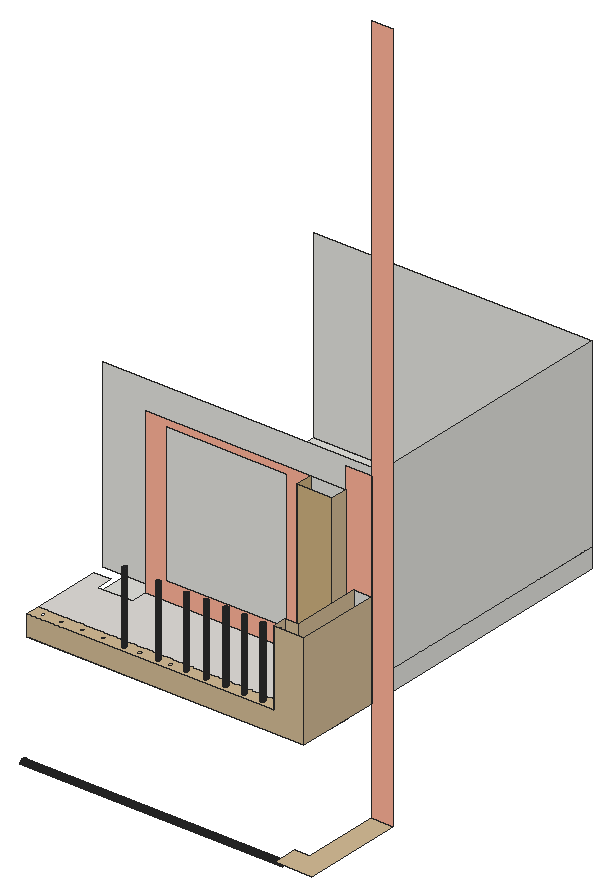
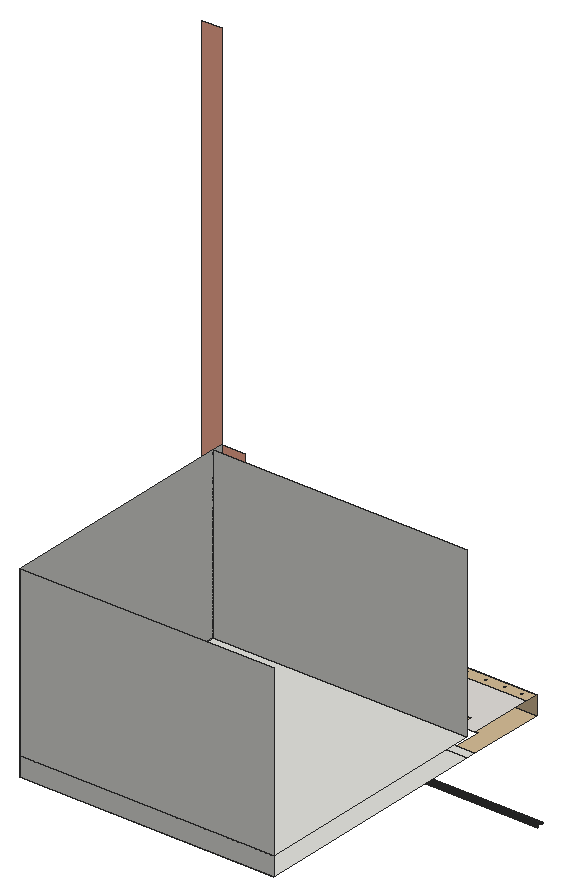
# SketchUp Ruby script. Lengths in inches.
U = 1.inch
M = Sketchup.active_model
def pt(a) = Geom::Point3d.new(a.map { |v| v * U })
def face(e, loops, mat)
  f = e.add_face(loops[0].map { |a| pt(a) })
  loops[1..].each { |l| e.add_face(l.map { |a| pt(a) }).erase! }
  f.material = f.back_material = mat if mat
  f
end
# faces: each face lists its corners as indices into pts; further lists are holes
def faces(e, pts, list, mat = nil) = list.each { |f| face(e, (f[0].is_a?(Array) ? f : [f]).map { |l| l.map { |i| pts[i] } }, mat) }
# xy, xz, yz: faces in a plane at the given z, y or x. An outline is a flat list of corners, or four numbers for a rectangle; further outlines are holes
def ring(l) = l.size == 4 ? [[l[0], l[1]], [l[2], l[1]], [l[2], l[3]], [l[0], l[3]]] : l.each_slice(2).to_a
def flat(e, list, mat, &to3) = list.each { |f| face(e, (f[0].is_a?(Array) ? f : [f]).map { |l| ring(l).map { |u, v| to3.(u, v) } }, mat) }
def xy(e, z, list, mat = nil) = flat(e, list, mat) { |x, y| [x, y, z] }
def xz(e, y, list, mat = nil) = flat(e, list, mat) { |x, z| [x, y, z] }
def yz(e, x, list, mat = nil) = flat(e, list, mat) { |y, z| [x, y, z] }
def lines(e, pts, list) = list.each { |a, b| e.add_line(pt(pts[a]), pt(pts[b])) }
# prism: a flat outline (further loops are holes) pulled along v
def prism(e, loops, v, mat = nil)
  f = face(e, loops, mat); d = Geom::Vector3d.new(v.map { |x| x * U })
  f.pushpull(f.normal.samedirection?(d) ? d.length : -d.length)
end
def box(e, o, s, mat = nil) = prism(e, [[o, [o[0] + s[0], o[1], o[2]], [o[0] + s[0], o[1] + s[1], o[2]], [o[0], o[1] + s[1], o[2]]]], [0, 0, s[2]], mat)
def at(x, y, z, deg = 0) = Geom::Transformation.translation(pt([x, y, z])) * Geom::Transformation.rotation(ORIGIN, Z_AXIS, deg.degrees)
def axes(o, x, y, z) = Geom::Transformation.new([*x, 0, *y, 0, *z, 0, *pt(o).to_a, 1])
def part(name) = M.definitions.add(name)
# library, detail: a bought-in or finely detailed component or shape, given as its bounding box
def library(name, o, s) = part(name).tap { |d| box(d.entities, o, s) }
def detail(e, o, s) = box(e.add_group.entities, o, s)
def put(e, d, t, mat = nil) = e.add_instance(d, t).tap { |i| i.material = mat if mat }
def group(e, t, mat = nil) = e.add_group.tap { |g| g.transformation = t; g.material = mat if mat }.entities
root = M.entities
M.materials.add("[Color B02]").color = [255, 178, 153]
M.materials.add("[Formica Beige]").color = [211, 187, 149]
M.materials.add("[Formica Laminate Dark]").color = [50, 53, 60]
M.materials.add("[Terrazzo Tile Accent]").color = [224, 221, 217]
M.materials.add("[Wood Floor Light]").color = [204, 176, 127]
xy(root,185.07,[[687.39,128.83,687.78,128.89,688.14,129.04,688.45,129.27,688.6875,129.58,688.84,129.95,688.89,130.33,688.84,130.72,688.6875,131.08,688.45,131.4,688.14,131.63,687.78,131.78,687.39,131.83,687,131.78,686.64,131.63,686.33,131.4,686.09,131.08,685.9375,130.72,685.89,130.33,685.9375,129.95,686.09,129.58,686.33,129.27,686.64,129.04,687,128.89]])
xy(root,189,[[765.67,122.79,786.87,122.79,786.87,182.57,774.15,182.57,774.15,137.11,765.67,137.11]],"[Formica Beige]")
xy(root,236.59,[[741.45,165.2,760.39,182.57]])
xy(root,236.59,[[641.83,165.2,741.45,182.57]],"[Wood Floor Light]")
xy(root,249,[[641.83,165.2,741.45,182.57],[741.45,165.2,760.39,182.57],[611.125,182.57,774.15,189.24],[611.125,189.24,774.15,344.36]])
xy(root,249,[[611.125,133.3,611.125,182.57,622.89,182.57,622.89,165.2,760.39,165.2,760.39,182.57,774.15,182.57,774.15,133.3]],"[Formica Beige]")
xy(root,261,[[665.36,136.16,665.06,136.2,664.77,136.32,664.52,136.51,664.34,136.76,664.22,137.04,664.18,137.35,664.22,137.66,664.34,137.94,664.52,138.19,664.77,138.38,665.06,138.5,665.36,138.54,665.67,138.5,665.96,138.38,666.2,138.19,666.39,137.94,666.51,137.66,666.55,137.35,666.51,137.04,666.39,136.76,666.2,136.51,665.96,136.32,665.67,136.2],[684.99,136.16,684.68,136.2,684.4,136.32,684.15,136.51,683.96,136.76,683.84,137.04,683.8,137.35,683.84,137.66,683.96,137.94,684.15,138.19,684.4,138.38,684.68,138.5,684.99,138.54,685.3,138.5,685.58,138.38,685.83,138.19,686.02,137.94,686.14,137.66,686.18,137.35,686.14,137.04,686.02,136.76,685.83,136.51,685.58,136.32,685.3,136.2],[701.43,136.16,701.12,136.2,700.83,136.32,700.59,136.51,700.4,136.76,700.28,137.04,700.24,137.35,700.28,137.66,700.4,137.94,700.59,138.19,700.83,138.38,701.12,138.5,701.43,138.54,701.73,138.5,702.02,138.38,702.27,138.19,702.46,137.94,702.57,137.66,702.61,137.35,702.57,137.04,702.46,136.76,702.27,136.51,702.02,136.32,701.73,136.2],[713.18,136.16,712.87,136.2,712.58,136.32,712.34,136.51,712.15,136.76,712.03,137.04,711.99,137.35,712.03,137.66,712.15,137.94,712.34,138.19,712.58,138.38,712.87,138.5,713.18,138.54,713.48,138.5,713.77,138.38,714.02,138.19,714.21,137.94,714.32,137.66,714.36,137.35,714.32,137.04,714.21,136.76,714.02,136.51,713.77,136.32,713.48,136.2],[724.8,136.16,724.49,136.2,724.21,136.32,723.96,136.51,723.77,136.76,723.66,137.04,723.61,137.35,723.66,137.66,723.77,137.94,723.96,138.19,724.21,138.38,724.49,138.5,724.8,138.54,725.11,138.5,725.4,138.38,725.64,138.19,725.83,137.94,725.95,137.66,725.99,137.35,725.95,137.04,725.83,136.76,725.64,136.51,725.4,136.32,725.11,136.2],
  [735.74,136.16,735.43,136.2,735.15,136.32,734.9,136.51,734.71,136.76,734.59,137.04,734.55,137.35,734.59,137.66,734.71,137.94,734.9,138.19,735.15,138.38,735.43,138.5,735.74,138.54,736.05,138.5,736.33,138.38,736.58,138.19,736.77,137.94,736.89,137.66,736.93,137.35,736.89,137.04,736.77,136.76,736.58,136.51,736.33,136.32,736.05,136.2],[746.55,136.16,746.24,136.2,745.96,136.32,745.71,136.51,745.52,136.76,745.41,137.04,745.36,137.35,745.41,137.66,745.52,137.94,745.71,138.19,745.96,138.38,746.24,138.5,746.55,138.54,746.86,138.5,747.15,138.38,747.39,138.19,747.58,137.94,747.7,137.66,747.74,137.35,747.7,137.04,747.58,136.76,747.39,136.51,747.15,136.32,746.86,136.2],[738.55,172.64,758.88,182.57],[611.125,189.24,774.15,344.36]])
xy(root,261,[[[611.125,133.3,755.9375,141.82],[692.47,135.92,692.13,135.96,691.82,136.09,691.55,136.3,691.34,136.57,691.21,136.89,691.16,137.23,691.21,137.57,691.34,137.88,691.55,138.16,691.82,138.36,692.13,138.5,692.47,138.54,692.8125,138.5,693.13,138.36,693.4,138.16,693.61,137.88,693.74,137.57,693.79,137.23,693.74,136.89,693.61,136.57,693.4,136.3,693.13,136.09,692.8125,135.96],[674.41,135.92,674.07,135.96,673.75,136.09,673.48,136.3,673.27,136.57,673.14,136.89,673.1,137.23,673.14,137.57,673.27,137.88,673.48,138.16,673.75,138.36,674.07,138.5,674.41,138.54,674.75,138.5,675.07,138.36,675.34,138.16,675.55,137.88,675.68,137.57,675.72,137.23,675.68,136.89,675.55,136.57,675.34,136.3,675.07,136.09,674.75,135.96],[617.36,136.16,617.06,136.2,616.77,136.32,616.52,136.51,616.34,136.76,616.22,137.04,616.18,137.35,616.22,137.66,616.34,137.94,616.52,138.19,616.77,138.38,617.06,138.5,617.36,138.54,617.67,138.5,617.96,138.38,618.2,138.19,618.39,137.94,618.51,137.66,618.55,137.35,618.51,137.04,618.39,136.76,618.2,136.51,617.96,136.32,617.67,136.2],[735.74,136.16,735.43,136.2,735.15,136.32,734.9,136.51,734.71,136.76,734.59,137.04,734.55,137.35,734.59,137.66,734.71,137.94,734.9,138.19,735.15,138.38,735.43,138.5,735.74,138.54,736.05,138.5,736.33,138.38,736.58,138.19,736.77,137.94,736.89,137.66,736.93,137.35,736.89,137.04,736.77,136.76,736.58,136.51,736.33,136.32,736.05,136.2],[628.3,136.16,627.99,136.2,627.71,136.32,627.46,136.51,627.27,136.76,627.16,137.04,627.11,137.35,627.16,137.66,627.27,137.94,627.46,138.19,627.71,138.38,627.99,138.5,628.3,138.54,628.61,138.5,628.9,138.38,629.14,138.19,629.33,137.94,629.45,137.66,629.49,137.35,629.45,137.04,629.33,136.76,629.14,136.51,628.9,136.32,628.61,136.2],[724.8,136.16,724.49,136.2,724.21,136.32,723.96,136.51,723.77,136.76,723.66,137.04,723.61,137.35,723.66,137.66,723.77,137.94,723.96,138.19,724.21,138.38,724.49,138.5,724.8,138.54,725.11,138.5,725.4,138.38,725.64,138.19,725.83,137.94,725.95,137.66,725.99,137.35,725.95,137.04,725.83,136.76,725.64,136.51,725.4,136.32,725.11,136.2],[640.36,136.16,640.06,136.2,639.77,136.32,639.52,136.51,639.34,136.76,639.22,137.04,639.18,137.35,639.22,137.66,639.34,137.94,639.52,138.19,639.77,138.38,640.06,138.5,640.36,138.54,640.67,138.5,640.96,138.38,641.2,138.19,641.39,137.94,641.51,137.66,641.55,137.35,641.51,137.04,641.39,136.76,641.2,136.51,640.96,136.32,640.67,136.2],[713.18,136.16,712.87,136.2,712.58,136.32,712.34,136.51,712.15,136.76,712.03,137.04,711.99,137.35,712.03,137.66,712.15,137.94,712.34,138.19,712.58,138.38,712.87,138.5,713.18,138.54,713.48,138.5,713.77,138.38,714.02,138.19,714.21,137.94,714.32,137.66,714.36,137.35,714.32,137.04,714.21,136.76,714.02,136.51,713.77,136.32,713.48,136.2],[652.55,136.16,652.24,136.2,651.96,136.32,651.71,136.51,651.52,136.76,651.41,137.04,651.36,137.35,651.41,137.66,651.52,137.94,651.71,138.19,651.96,138.38,652.24,138.5,652.55,138.54,652.86,138.5,653.15,138.38,653.39,138.19,653.58,137.94,653.7,137.66,653.74,137.35,653.7,137.04,653.58,136.76,653.39,136.51,653.15,136.32,652.86,136.2],[701.43,136.16,701.12,136.2,700.83,136.32,700.59,136.51,700.4,136.76,700.28,137.04,700.24,137.35,700.28,137.66,700.4,137.94,700.59,138.19,700.83,138.38,701.12,138.5,701.43,138.54,701.73,138.5,702.02,138.38,702.27,138.19,702.46,137.94,702.57,137.66,702.61,137.35,702.57,137.04,702.46,136.76,702.27,136.51,702.02,136.32,701.73,136.2],[665.36,136.16,665.06,136.2,664.77,136.32,664.52,136.51,664.34,136.76,664.22,137.04,664.18,137.35,664.22,137.66,664.34,137.94,664.52,138.19,664.77,138.38,665.06,138.5,665.36,138.54,665.67,138.5,665.96,138.38,666.2,138.19,666.39,137.94,666.51,137.66,666.55,137.35,666.51,137.04,666.39,136.76,666.2,136.51,665.96,136.32,665.67,136.2],[684.99,136.16,684.68,136.2,684.4,136.32,684.15,136.51,683.96,136.76,683.84,137.04,683.8,137.35,683.84,137.66,683.96,137.94,684.15,138.19,684.4,138.38,684.68,138.5,684.99,138.54,685.3,138.5,685.58,138.38,685.83,138.19,686.02,137.94,686.14,137.66,686.18,137.35,686.14,137.04,686.02,136.76,685.83,136.51,685.58,136.32,685.3,136.2],[746.55,136.16,746.24,136.2,745.96,136.32,745.71,136.51,745.52,136.76,745.41,137.04,745.36,137.35,745.41,137.66,745.52,137.94,745.71,138.19,745.96,138.38,746.24,138.5,746.55,138.54,746.86,138.5,747.15,138.38,747.39,138.19,747.58,137.94,747.7,137.66,747.74,137.35,747.7,137.04,747.58,136.76,747.39,136.51,747.15,136.32,746.86,136.2]]],"[Formica Beige]")
xy(root,261,[[611.125,141.82,764,141.82,764,182.57,758.88,182.57,758.88,172.64,738.55,172.64,738.55,182.57,641.63,182.57,641.63,172.64,621.3,172.64,621.3,182.57,611.125,182.57]],"[Terrazzo Tile Accent]")
xz(root,133.3,[[611.125,249,774.15,249,774.15,305.625,755.9375,305.625,755.9375,261,611.125,261]],"[Formica Beige]")
xz(root,141.82,[[755.9375,261,764,305.625]],"[Formica Beige]")
xz(root,165.2,[[641.83,236.59,741.45,249],[741.45,236.59,760.39,249]],"[Wood Floor Light]")
xz(root,172.64,[[738.55,261,758.88,356.625]],"[Wood Floor Light]")
xz(root,182.57,[[641.83,236.59,741.45,249],[741.45,236.59,760.39,249],[738.55,261,758.88,356.625]])
xz(root,182.57,[[774.15,189,786.87,609],[[641.63,261,738.55,356.625],[653.42,271.33,724.17,352.83]],[758.88,261,764,261,764,305.625,774.15,305.625,774.15,369,758.88,369]],"[Color B02]")
xz(root,189.24,[[611.125,261,774.15,369]])
xz(root,344.36,[[611.125,249,774.15,261],[611.125,261,774.15,369]])
yz(root,738.55,[[172.64,261,182.57,356.625]],"[Wood Floor Light]")
yz(root,741.45,[[165.2,236.59,182.57,249]])
yz(root,755.9375,[[[133.3,261,141.82,305.625],[138.08,300.72,138.39,300.77,138.68,300.88,138.92,301.07,139.11,301.32,139.23,301.6,139.27,301.91,139.23,302.22,139.11,302.51,138.92,302.75,138.68,302.94,138.39,303.06,138.08,303.1,137.78,303.06,137.49,302.94,137.25,302.75,137.06,302.51,136.9375,302.22,136.9,301.91,136.9375,301.6,137.06,301.32,137.25,301.07,137.49,300.88,137.78,300.77]]],"[Formica Beige]")
yz(root,758.88,[[172.64,261,182.57,356.625]],"[Formica Beige]")
yz(root,760.39,[[165.2,236.59,182.57,249]],"[Wood Floor Light]")
yz(root,764,[[141.82,261,182.57,305.625]],"[Formica Beige]")
yz(root,774.15,[[182.57,249,189.24,369],[189.24,249,344.36,261],[189.24,261,344.36,369]])
yz(root,774.15,[[133.3,249,182.57,305.625]],"[Formica Beige]")
p = [[765.67,128.24,184.07],[765.67,128.3125,184.59],[611.125,128.3125,184.59],[611.125,128.24,184.07],[765.67,132.18,184.59],[765.67,132.24,184.07],
  [611.125,132.24,184.07],[611.125,132.18,184.59],[765.67,128.51,185.07],[611.125,128.51,185.07],[765.67,131.98,185.07],[611.125,131.98,185.07],
  [765.67,128.83,185.49],[611.125,128.83,185.49],[765.67,131.66,185.49],[611.125,131.66,185.49],[765.67,129.24,185.8],[611.125,129.24,185.8],
  [765.67,131.24,185.8],[611.125,131.24,185.8],[765.67,129.73,186],[611.125,129.73,186],[765.67,130.76,186],[611.125,130.76,186],
  [765.67,130.24,186.07],[611.125,130.24,186.07],[664.77,136.32,261],[665.06,136.2,261],[665.06,136.2,302.8125],[664.77,136.32,302.8125],
  [665.36,136.16,261],[665.36,136.16,302.8125],[665.67,136.2,261],[665.67,136.2,302.8125],[665.96,136.32,261],[665.96,136.32,302.8125],
  [684.4,136.32,261],[684.68,136.2,261],[684.68,136.2,302.125],[684.4,136.32,302.125],[684.99,136.16,261],[684.99,136.16,302.125],
  [685.3,136.2,261],[685.3,136.2,302.125],[685.58,136.32,261],[685.58,136.32,302.125],[700.83,136.32,261],[701.12,136.2,261],
  [701.12,136.2,301.9375],[700.83,136.32,301.9375],[701.43,136.16,261],[701.43,136.16,301.9375],[701.73,136.2,261],[701.73,136.2,301.9375],
  [702.02,136.32,261],[702.02,136.32,301.9375],[712.58,136.32,261],[712.87,136.2,261],[712.87,136.2,302.3125],[712.58,136.32,302.3125],
  [713.18,136.16,261],[713.18,136.16,302.3125],[713.48,136.2,261],[713.48,136.2,302.3125],[713.77,136.32,261],[713.77,136.32,302.3125],
  [724.21,136.32,261],[724.49,136.2,261],[724.49,136.2,302.375],[724.21,136.32,302.375],[724.8,136.16,261],[724.8,136.16,302.375],
  [725.11,136.2,261],[725.11,136.2,302.375],[725.4,136.32,261],[725.4,136.32,302.375],[735.15,136.32,261],[735.43,136.2,261],
  [735.43,136.2,302.1875],[735.15,136.32,302.1875],[735.74,136.16,261],[735.74,136.16,302.1875],[736.05,136.2,261],[736.05,136.2,302.1875],
  [736.33,136.32,261],[736.33,136.32,302.1875],[745.96,136.32,261],[746.24,136.2,261],[746.24,136.2,301.875],[745.96,136.32,301.875],
  [746.55,136.16,261],[746.55,136.16,301.875],[746.86,136.2,261],[746.86,136.2,301.875],[747.15,136.32,261],[747.15,136.32,301.875],
  [664.52,136.51,261],[664.52,136.51,302.8125],[666.2,136.51,261],[666.2,136.51,302.8125],[684.15,136.51,261],[684.15,136.51,302.125],
  [685.83,136.51,261],[685.83,136.51,302.125],[700.59,136.51,261],[700.59,136.51,301.9375],[702.27,136.51,261],[702.27,136.51,301.9375],
  [712.34,136.51,261],[712.34,136.51,302.3125],[714.02,136.51,261],[714.02,136.51,302.3125],[723.96,136.51,261],[723.96,136.51,302.375],
  [725.64,136.51,261],[725.64,136.51,302.375],[734.9,136.51,261],[734.9,136.51,302.1875],[736.58,136.51,261],[736.58,136.51,302.1875],
  [745.71,136.51,261],[745.71,136.51,301.875],[747.39,136.51,261],[747.39,136.51,301.875],[664.34,136.76,261],[664.34,136.76,302.8125],
  [666.39,136.76,261],[666.39,136.76,302.8125],[683.96,136.76,261],[683.96,136.76,302.125],[686.02,136.76,261],[686.02,136.76,302.125],
  [700.4,136.76,261],[700.4,136.76,301.9375],[702.46,136.76,261],[702.46,136.76,301.9375],[712.15,136.76,261],[712.15,136.76,302.3125],
  [714.21,136.76,261],[714.21,136.76,302.3125],[723.77,136.76,261],[723.77,136.76,302.375],[725.83,136.76,261],[725.83,136.76,302.375],
  [734.71,136.76,261],[734.71,136.76,302.1875],[736.77,136.76,261],[736.77,136.76,302.1875],[745.52,136.76,261],[745.52,136.76,301.875],
  [747.58,136.76,261],[747.58,136.76,301.875],[666.51,137.04,261],[666.51,137.04,302.8125],[683.84,137.04,261],[683.84,137.04,302.125],
  [686.14,137.04,261],[686.14,137.04,302.125],[700.28,137.04,261],[700.28,137.04,301.9375],[702.57,137.04,261],[702.57,137.04,301.9375],
  [712.03,137.04,261],[712.03,137.04,302.3125],[714.32,137.04,261],[714.32,137.04,302.3125],[723.66,137.04,261],[723.66,137.04,302.375],
  [725.95,137.04,261],[725.95,137.04,302.375],[734.59,137.04,261],[734.59,137.04,302.1875],[736.89,137.04,261],[736.89,137.04,302.1875],
  [745.41,137.04,261],[745.41,137.04,301.875],[747.7,137.04,261],[747.7,137.04,301.875],[666.55,137.35,261],[666.55,137.35,302.8125],
  [683.8,137.35,261],[683.8,137.35,302.125],[686.18,137.35,261],[686.18,137.35,302.125],[700.24,137.35,261],[700.24,137.35,301.9375],
  [702.61,137.35,261],[702.61,137.35,301.9375],[711.99,137.35,261],[711.99,137.35,302.3125],[714.36,137.35,261],[714.36,137.35,302.3125],
  [723.61,137.35,261],[723.61,137.35,302.375],[725.99,137.35,261],[725.99,137.35,302.375],[734.55,137.35,261],[734.55,137.35,302.1875],
  [736.93,137.35,261],[736.93,137.35,302.1875],[745.36,137.35,261],[745.36,137.35,301.875],[747.74,137.35,261],[747.74,137.35,301.875],
  [666.51,137.66,261],[666.51,137.66,302.8125],[683.84,137.66,261],[683.84,137.66,302.125],[686.14,137.66,261],[686.14,137.66,302.125],
  [700.28,137.66,261],[700.28,137.66,301.9375],[702.57,137.66,261],[702.57,137.66,301.9375],[712.03,137.66,261],[712.03,137.66,302.3125],
  [714.32,137.66,261],[714.32,137.66,302.3125],[723.66,137.66,261],[723.66,137.66,302.375],[725.95,137.66,261],[725.95,137.66,302.375],
  [734.59,137.66,261],[734.59,137.66,302.1875],[736.89,137.66,261],[736.89,137.66,302.1875],[745.41,137.66,261],[745.41,137.66,301.875],
  [747.7,137.66,261],[747.7,137.66,301.875],[666.39,137.94,261],[666.39,137.94,302.8125],[683.96,137.94,261],[683.96,137.94,302.125],
  [686.02,137.94,261],[686.02,137.94,302.125],[700.4,137.94,261],[700.4,137.94,301.9375],[702.46,137.94,261],[702.46,137.94,301.9375],
  [712.15,137.94,261],[712.15,137.94,302.3125],[714.21,137.94,261],[714.21,137.94,302.3125],[723.77,137.94,261],[723.77,137.94,302.375],
  [725.83,137.94,261],[725.83,137.94,302.375],[734.71,137.94,261],[734.71,137.94,302.1875],[736.77,137.94,261],[736.77,137.94,302.1875],
  [745.52,137.94,261],[745.52,137.94,301.875],[747.58,137.94,261],[747.58,137.94,301.875],[664.52,138.19,261],[664.34,137.94,261],
  [664.34,137.94,302.8125],[664.52,138.19,302.8125],[666.2,138.19,261],[666.2,138.19,302.8125],[684.15,138.19,261],[684.15,138.19,302.125],
  [685.83,138.19,261],[685.83,138.19,302.125],[700.59,138.19,261],[700.59,138.19,301.9375],[702.27,138.19,261],[702.27,138.19,301.9375],
  [712.34,138.19,261],[712.34,138.19,302.3125],[714.02,138.19,261],[714.02,138.19,302.3125],[723.96,138.19,261],[723.96,138.19,302.375],
  [725.64,138.19,261],[725.64,138.19,302.375],[734.9,138.19,261],[734.9,138.19,302.1875],[736.58,138.19,261],[736.58,138.19,302.1875],
  [745.71,138.19,261],[745.71,138.19,301.875],[747.39,138.19,261],[747.39,138.19,301.875],[664.77,138.38,261],[664.77,138.38,302.8125],
  [665.96,138.38,261],[665.96,138.38,302.8125],[684.4,138.38,261],[684.4,138.38,302.125],[685.58,138.38,261],[685.58,138.38,302.125],
  [700.83,138.38,261],[700.83,138.38,301.9375],[702.02,138.38,261],[702.02,138.38,301.9375],[712.58,138.38,261],[712.58,138.38,302.3125],
  [713.77,138.38,261],[713.77,138.38,302.3125],[724.21,138.38,261],[724.21,138.38,302.375],[725.4,138.38,261],[725.4,138.38,302.375],
  [735.15,138.38,261],[735.15,138.38,302.1875],[736.33,138.38,261],[736.33,138.38,302.1875],[745.96,138.38,261],[745.96,138.38,301.875],
  [747.15,138.38,261],[747.15,138.38,301.875],[665.06,138.5,261],[665.06,138.5,302.8125],[665.67,138.5,261],[665.67,138.5,302.8125],
  [684.68,138.5,261],[684.68,138.5,302.125],[685.3,138.5,261],[685.3,138.5,302.125],[701.12,138.5,261],[701.12,138.5,301.9375],
  [701.73,138.5,261],[701.73,138.5,301.9375],[712.87,138.5,261],[712.87,138.5,302.3125],[713.48,138.5,261],[713.48,138.5,302.3125],
  [724.49,138.5,261],[724.49,138.5,302.375],[725.11,138.5,261],[725.11,138.5,302.375],[735.43,138.5,261],[735.43,138.5,302.1875],
  [736.05,138.5,261],[736.05,138.5,302.1875],[746.24,138.5,261],[746.24,138.5,301.875],[746.86,138.5,261],[746.86,138.5,301.875],
  [665.36,138.54,261],[665.36,138.54,302.8125],[684.99,138.54,261],[684.99,138.54,302.125],[701.43,138.54,261],[701.43,138.54,301.9375],
  [713.18,138.54,261],[713.18,138.54,302.3125],[724.8,138.54,261],[724.8,138.54,302.375],[735.74,138.54,261],[735.74,138.54,302.1875],
  [746.55,138.54,261],[746.55,138.54,301.875]]
faces(root,p,[[0,1,2,3],[4,5,6,7],[1,8,9,2],[10,4,7,11],[8,12,13,9],[14,10,11,15],[12,16,17,13],[18,14,15,19],
  [16,20,21,17],[22,18,19,23],[20,24,25,21],[24,22,23,25],[26,27,28,29],[27,30,31,28],[30,32,33,31],[32,34,35,33],
  [36,37,38,39],[37,40,41,38],[40,42,43,41],[42,44,45,43],[46,47,48,49],[47,50,51,48],[50,52,53,51],[52,54,55,53],
  [56,57,58,59],[57,60,61,58],[60,62,63,61],[62,64,65,63],[66,67,68,69],[67,70,71,68],[70,72,73,71],[72,74,75,73],
  [76,77,78,79],[77,80,81,78],[80,82,83,81],[82,84,85,83],[86,87,88,89],[87,90,91,88],[90,92,93,91],[92,94,95,93],
  [96,26,29,97],[34,98,99,35],[100,36,39,101],[44,102,103,45],[104,46,49,105],[54,106,107,55],[108,56,59,109],[64,110,111,65],
  [112,66,69,113],[74,114,115,75],[116,76,79,117],[84,118,119,85],[120,86,89,121],[94,122,123,95],[124,96,97,125],[98,126,127,99],
  [128,100,101,129],[102,130,131,103],[132,104,105,133],[106,134,135,107],[136,108,109,137],[110,138,139,111],[140,112,113,141],[114,142,143,115],
  [144,116,117,145],[118,146,147,119],[148,120,121,149],[122,150,151,123],[126,152,153,127],[154,128,129,155],[130,156,157,131],[158,132,133,159],
  [134,160,161,135],[162,136,137,163],[138,164,165,139],[166,140,141,167],[142,168,169,143],[170,144,145,171],[146,172,173,147],[174,148,149,175],
  [150,176,177,151],[152,178,179,153],[180,154,155,181],[156,182,183,157],[184,158,159,185],[160,186,187,161],[188,162,163,189],[164,190,191,165],
  [192,166,167,193],[168,194,195,169],[196,170,171,197],[172,198,199,173],[200,174,175,201],[176,202,203,177],[178,204,205,179],[206,180,181,207],
  [182,208,209,183],[210,184,185,211],[186,212,213,187],[214,188,189,215],[190,216,217,191],[218,192,193,219],[194,220,221,195],[222,196,197,223],
  [198,224,225,199],[226,200,201,227],[202,228,229,203],[204,230,231,205],[232,206,207,233],[208,234,235,209],[236,210,211,237],[212,238,239,213],
  [240,214,215,241],[216,242,243,217],[244,218,219,245],[220,246,247,221],[248,222,223,249],[224,250,251,225],[252,226,227,253],[228,254,255,229],
  [256,257,258,259],[230,260,261,231],[262,232,233,263],[234,264,265,235],[266,236,237,267],[238,268,269,239],[270,240,241,271],[242,272,273,243],
  [274,244,245,275],[246,276,277,247],[278,248,249,279],[250,280,281,251],[282,252,253,283],[254,284,285,255],[286,256,259,287],[260,288,289,261],
  [290,262,263,291],[264,292,293,265],[294,266,267,295],[268,296,297,269],[298,270,271,299],[272,300,301,273],[302,274,275,303],[276,304,305,277],
  [306,278,279,307],[280,308,309,281],[310,282,283,311],[284,312,313,285],[314,286,287,315],[288,316,317,289],[318,290,291,319],[292,320,321,293],
  [322,294,295,323],[296,324,325,297],[326,298,299,327],[300,328,329,301],[330,302,303,331],[304,332,333,305],[334,306,307,335],[308,336,337,309],
  [338,310,311,339],[312,340,341,313],[342,314,315,343],[316,342,343,317],[344,318,319,345],[320,344,345,321],[346,322,323,347],[324,346,347,325],
  [348,326,327,349],[328,348,349,329],[350,330,331,351],[332,350,351,333],[352,334,335,353],[336,352,353,337],[354,338,339,355],[340,354,355,341]],"[Formica Laminate Dark]")
